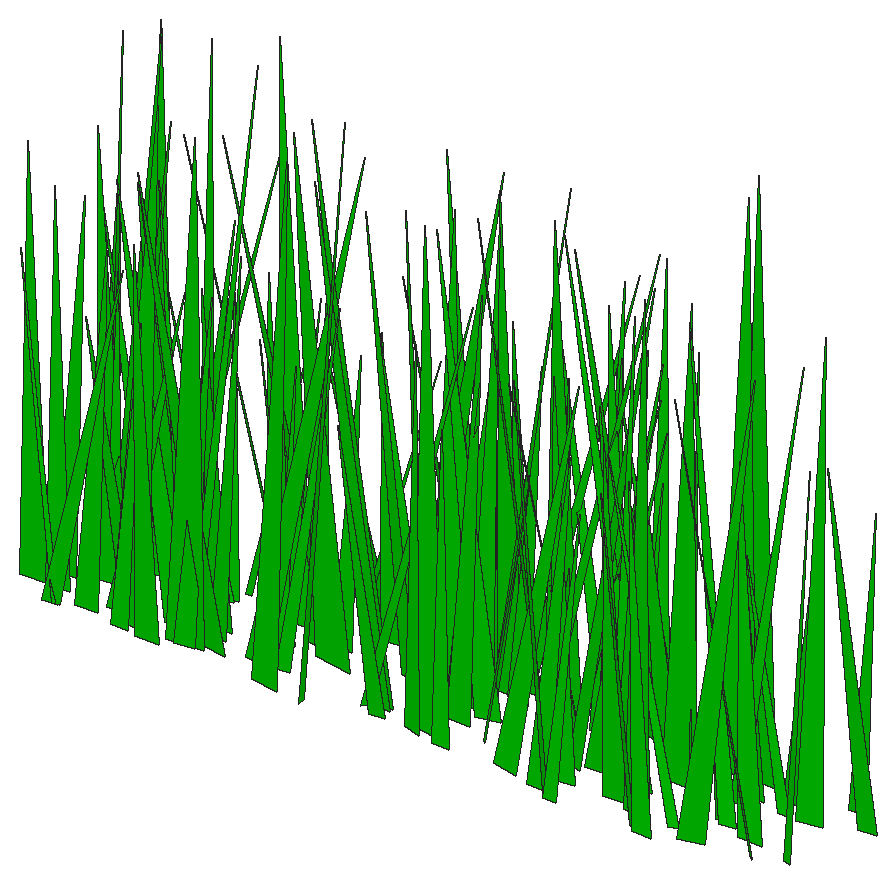
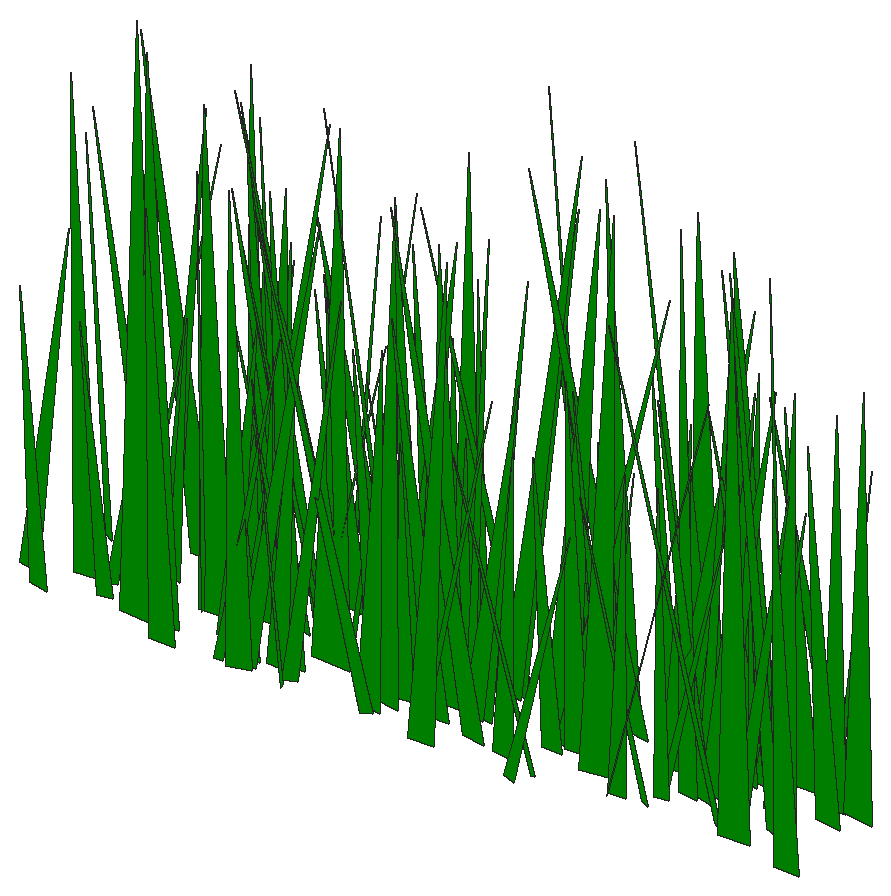
# SketchUp Ruby script. Lengths in inches.
U = 1.inch
M = Sketchup.active_model
def pt(a) = Geom::Point3d.new(a.map { |v| v * U })
def face(e, loops, mat)
  f = e.add_face(loops[0].map { |a| pt(a) })
  loops[1..].each { |l| e.add_face(l.map { |a| pt(a) }).erase! }
  f.material = f.back_material = mat if mat
  f
end
# faces: each face lists its corners as indices into pts; further lists are holes
def faces(e, pts, list, mat = nil) = list.each { |f| face(e, (f[0].is_a?(Array) ? f : [f]).map { |l| l.map { |i| pts[i] } }, mat) }
# xy, xz, yz: faces in a plane at the given z, y or x. An outline is a flat list of corners, or four numbers for a rectangle; further outlines are holes
def ring(l) = l.size == 4 ? [[l[0], l[1]], [l[2], l[1]], [l[2], l[3]], [l[0], l[3]]] : l.each_slice(2).to_a
def flat(e, list, mat, &to3) = list.each { |f| face(e, (f[0].is_a?(Array) ? f : [f]).map { |l| ring(l).map { |u, v| to3.(u, v) } }, mat) }
def xy(e, z, list, mat = nil) = flat(e, list, mat) { |x, y| [x, y, z] }
def xz(e, y, list, mat = nil) = flat(e, list, mat) { |x, z| [x, y, z] }
def yz(e, x, list, mat = nil) = flat(e, list, mat) { |y, z| [x, y, z] }
def lines(e, pts, list) = list.each { |a, b| e.add_line(pt(pts[a]), pt(pts[b])) }
# prism: a flat outline (further loops are holes) pulled along v
def prism(e, loops, v, mat = nil)
  f = face(e, loops, mat); d = Geom::Vector3d.new(v.map { |x| x * U })
  f.pushpull(f.normal.samedirection?(d) ? d.length : -d.length)
end
def box(e, o, s, mat = nil) = prism(e, [[o, [o[0] + s[0], o[1], o[2]], [o[0] + s[0], o[1] + s[1], o[2]], [o[0], o[1] + s[1], o[2]]]], [0, 0, s[2]], mat)
def at(x, y, z, deg = 0) = Geom::Transformation.translation(pt([x, y, z])) * Geom::Transformation.rotation(ORIGIN, Z_AXIS, deg.degrees)
def axes(o, x, y, z) = Geom::Transformation.new([*x, 0, *y, 0, *z, 0, *pt(o).to_a, 1])
def part(name) = M.definitions.add(name)
# library, detail: a bought-in or finely detailed component or shape, given as its bounding box
def library(name, o, s) = part(name).tap { |d| box(d.entities, o, s) }
def detail(e, o, s) = box(e.add_group.entities, o, s)
def put(e, d, t, mat = nil) = e.add_instance(d, t).tap { |i| i.material = mat if mat }
def group(e, t, mat = nil) = e.add_group.tap { |g| g.transformation = t; g.material = mat if mat }.entities
root = M.entities
M.materials.add("[Color G06]").color = [0, 204, 0]
c1 = part("fur_instance\#9")
p = [[0.8125,0,1.79],[0.67,-0.02,1.48],[0,-0.11,0],[0,0.11,0]]
faces(c1.entities,p,[[0,1,2,3]])
put(root,c1,axes([66.83,16.76,4.28],[0.70712,0.57146,2.51292],[4.40533,-0.11555,0.24948],[-0.46309,-0.22659,6.2104]),"[Color G06]")
put(root,c1,axes([66.57,20.13,4.28],[1.66976,-0.51159,0.9789],[-3.70784,-0.23812,-0.16793],[-0.37482,0.07652,6.02204]),"[Color G06]")
put(root,c1,axes([68.1,16.04,4.28],[-3.45503,0.0613,1.28299],[0.39453,0.4961,-0.34967],[0.88006,0.01826,5.19367]),"[Color G06]")
put(root,c1,axes([67.29,17.46,4.28],[1.39054,0.5281,0.88835],[3.81428,-0.19942,0.2814],[-0.3833,-0.06857,6.02306]),"[Color G06]")
put(root,c1,axes([67.625,16.76,4.28],[-2.06098,0.45345,2.2384],[3.47569,0.3112,-0.0935],[0.85835,-0.17136,5.75321]),"[Color G06]")
put(root,c1,axes([68.6,17.85,4.28],[-0.6422,0.67546,0.37884],[4.84661,0.08792,0.34379],[-0.19506,-0.03922,7.29482]),"[Color G06]")
put(root,c1,axes([69.18,18.85,4.28],[-3.10384,0.27643,0.94882],[2.03869,0.43579,0.31188],[0.42019,-0.07246,5.49549]),"[Color G06]")
put(root,c1,axes([68.12,18.32,4.28],[5.07652,0.17543,3.19542],[1.41724,-0.76243,-0.22092],[-2.036,-0.0933,7.81363]),"[Color G06]")
put(root,c1,axes([68.54,17.97,4.28],[-1.98125,0.30032,1.94706],[2.31896,0.30769,-0.18089],[0.97875,-0.12107,4.36994]),"[Color G06]")
put(root,c1,axes([68.08,18.76,4.28],[4.81626,0.3761,2.3505],[2.78245,-0.69993,0.12995],[-1.41619,-0.09614,8.24905]),"[Color G06]")
put(root,c1,axes([68.7,19.68,4.28],[-1.91202,-0.68423,2.93449],[-5.19419,0.29703,0.39628],[0.97564,0.24046,7.86064]),"[Color G06]")
put(root,c1,axes([67.97,16.03,4.28],[3.31947,-0.34025,0.11832],[-2.4411,-0.46283,0.08668],[-0.02942,0.01305,6.15668]),"[Color G06]")
put(root,c1,axes([69.99,16.875,4.28],[-1.54754,-0.3765,0.40529],[-2.71341,0.21421,-0.284],[-0.03089,0.04597,4.64251]),"[Color G06]")
put(root,c1,axes([68.92,16.34,4.28],[1.95061,-0.46199,1.20205],[-3.38606,-0.27757,0.01875],[-0.39701,0.09755,5.74603]),"[Color G06]")
put(root,c1,axes([70.57,18.18,4.28],[-1.25331,-0.60584,0.50701],[-4.35782,0.17399,-0.17996],[-0.02202,0.0501,6.75578]),"[Color G06]")
put(root,c1,axes([71.33,17.18,4.28],[-3.00174,0.47818,0.48813],[3.44352,0.41813,0.24732],[0.09014,-0.04948,6.80686]),"[Color G06]")
put(root,c1,axes([70.125,17.08,4.28],[2.45799,-0.13614,1.39658],[-0.94327,-0.36651,-0.39592],[-0.96778,0.01145,3.93296]),"[Color G06]")
put(root,c1,axes([69.69,16.93,4.28],[4.64119,0.29399,2.06947],[2.19856,-0.66971,-0.08469],[-1.23632,-0.08731,7.61827]),"[Color G06]")
put(root,c1,axes([71.68,19,4.28],[-3.04482,0.11833,0.27712],[0.85341,0.42509,0.0941],[0.16164,-0.01541,4.72318]),"[Color G06]")
put(root,c1,axes([70.22,16.12,4.28],[2.28875,-0.28835,1.54865],[-2.22991,-0.32907,0.32314],[-0.61407,0.12023,4.59871]),"[Color G06]")
put(root,c1,axes([70.4,16.36,4.28],[0.41336,0.76781,1.30806],[5.57291,-0.05332,-0.33883],[0.16343,-0.12399,8.24559]),"[Color G06]")
put(root,c1,axes([69.57,16.8,4.28],[3.12255,-0.33232,0.11448],[-2.38433,-0.43528,0.12169],[-0.01147,0.01551,5.8695]),"[Color G06]")
put(root,c1,axes([71.23,16.02,4.28],[-1.27828,-0.49619,2.17206],[-3.82734,0.18396,-0.20394],[0.35344,0.19749,5.64718]),"[Color G06]")
put(root,c1,axes([72.89,19.86,4.28],[-4.76011,-0.05072,0.37207],[-0.35967,0.66462,0.12951],[0.25479,-0.00942,7.13391]),"[Color G06]")
put(root,c1,axes([69.45,19.4,4.28],[4.95223,0.23128,0.28465],[1.64836,-0.69056,0.39613],[-0.26459,0.02665,7.79548]),"[Color G06]")
put(root,c1,axes([71.15,18.57,4.28],[4.44586,0.42134,3.46668],[3.31303,-0.67304,-0.09391],[-1.87979,-0.18969,8.03344]),"[Color G06]")
put(root,c1,axes([70.68,18.49,4.28],[2.95516,0.40171,0.98328],[2.89801,-0.41935,0.22517],[-0.57728,-0.04876,6.16395]),"[Color G06]")
put(root,c1,axes([72.17,16.57,4.28],[-4.27976,0.16657,2.23807],[1.29906,0.62802,0.17965],[1.40771,-0.07315,6.63845]),"[Color G06]")
put(root,c1,axes([71.625,19.125,4.28],[2.29948,-0.25988,1.81629],[-2.00537,-0.34765,-0.0431],[-0.96369,0.10332,4.42357]),"[Color G06]")
put(root,c1,axes([72.97,16.66,4.28],[-3.17325,-0.55502,0.35688],[-3.9826,0.44325,0.08797],[0.19492,0.02091,7.60738]),"[Color G06]")
put(root,c1,axes([72.35,17.69,4.28],[-0.24066,-0.53785,0.10636],[-3.85756,0.03345,-0.06409],[-0.03838,0.01028,5.77556]),"[Color G06]")
put(root,c1,axes([72.66,19.74,4.28],[-2.08194,0.32799,1.85752],[2.54477,0.30969,0.08937],[0.77544,-0.13569,4.69386]),"[Color G06]")
put(root,c1,axes([72.18,16.46,4.28],[1.4281,-0.80026,0.17463],[-5.73713,-0.19954,-0.23835],[-0.18299,0.01043,8.83551]),"[Color G06]")
put(root,c1,axes([72.2,16.4,4.28],[2.43363,-0.406,1.10403],[-2.96298,-0.34625,-0.03765],[-0.49343,0.07674,5.6713]),"[Color G06]")
put(root,c1,axes([71.8,19.625,4.28],[2.9454,0.17528,0.18578],[1.24841,-0.41066,0.29747],[-0.19229,0.01876,4.77698]),"[Color G06]")
put(root,c1,axes([72.62,17.29,4.28],[2.6975,0.39177,1.63323],[2.89485,-0.3937,0.16868],[-0.84107,-0.09855,5.81871]),"[Color G06]")
put(root,c1,axes([72.06,16.94,4.28],[6.03467,-0.12505,2.2423],[-0.92586,-0.86653,0.01481],[-1.4825,0.03216,9.11829]),"[Color G06]")
put(root,c1,axes([73.81,19.19,4.28],[-3.29736,0.66619,2.36389],[4.92298,0.4817,-0.25527],[1.04374,-0.16742,8.67199]),"[Color G06]")
put(root,c1,axes([75.51,18.51,4.28],[-4.78607,-0.3499,0.24867],[-2.50185,0.66756,0.34529],[0.25455,-0.01778,8.06924]),"[Color G06]")
put(root,c1,axes([74.37,18.27,4.28],[-2.78305,-0.16238,1.02207],[-1.16808,0.39908,0.17881],[0.67771,0.021,4.50537]),"[Color G06]")
put(root,c1,axes([74.34,17.85,4.28],[0.64409,-0.3519,1.03219],[-2.60627,-0.09499,-0.08755],[-0.22947,0.0912,3.89157]),"[Color G06]")
put(root,c1,axes([75.48,20.8,4.28],[-2.2374,-0.26843,0.12242],[-1.92497,0.31068,-0.33011],[-0.08219,0.03079,4.39891]),"[Color G06]")
put(root,c1,axes([74,18.4375,4.28],[3.44354,-0.17526,1.2215],[-1.23929,-0.49343,-0.32894],[-0.84368,0.00947,5.46883]),"[Color G06]")
put(root,c1,axes([74.45,17.625,4.28],[2.34333,-0.24978,1.31817],[-1.86168,-0.34187,-0.04904],[-0.72146,0.07089,4.408]),"[Color G06]")
put(root,c1,axes([74.93,18.59,4.28],[0.70413,0.48637,2.10076],[3.75822,-0.09787,-0.21083],[-0.12926,-0.19616,5.31386]),"[Color G06]")
put(root,c1,axes([75.91,18.05,4.28],[-1.93115,-0.76471,0.66967],[-5.48915,0.27232,0.36408],[0.37915,0.04757,8.68189]),"[Color G06]")
put(root,c1,axes([75.18,16.07,4.28],[-3.09751,-0.50765,4.07289],[-4.18001,0.49891,0.04245],[1.79081,0.28646,7.14383]),"[Color G06]")
put(root,c1,axes([75.52,18.91,4.28],[0.46261,0.44036,0.46927],[3.17326,-0.06365,-0.12606],[0.03836,-0.04502,4.76845]),"[Color G06]")
put(root,c1,axes([74.28,16.88,4.28],[4.42171,0.5679,0.29919],[4.07454,-0.61697,0.01815],[-0.15548,-0.01766,8.98453]),"[Color G06]")
put(root,c1,axes([75.0625,16.99,4.28],[3.69686,-0.2435,0.98505],[-1.78111,-0.5212,0.13095],[-0.55791,0.05043,6.10919]),"[Color G06]")
put(root,c1,axes([76.37,19.94,4.28],[0.1093,-0.41163,1.75668],[-3.1703,-0.025,-0.23224],[-0.21055,0.1627,4.40873]),"[Color G06]")
put(root,c1,axes([75.0625,20.29,4.28],[3.16739,0.1345,0.01271],[0.96247,-0.44044,-0.36675],[0.06337,-0.03308,4.93491]),"[Color G06]")
put(root,c1,axes([78.3,17.19,4.28],[-4.62122,-0.50231,1.73508],[-3.68936,0.65488,-0.17026],[0.84404,0.11228,8.75554]),"[Color G06]")
put(root,c1,axes([76.5,15.98,4.28],[5.92277,-0.007,2.76756],[-0.03278,-0.8653,-0.09468],[-1.85213,-0.00707,8.85183]),"[Color G06]")
put(root,c1,axes([78.25,17.08,4.28],[-3.75777,-0.52209,1.39761],[-3.81141,0.53063,-0.12025],[0.60469,0.1001,7.92721]),"[Color G06]")
put(root,c1,axes([77.95,18.72,4.28],[-3.90089,-0.35092,1.67875],[-2.55758,0.56209,0.22217],[1.02629,0.06694,6.93452]),"[Color G06]")
put(root,c1,axes([78.3,18.8125,4.28],[-2.59319,0.39094,0.74982],[2.83994,0.36208,0.25292],[0.21504,-0.06747,5.7021]),"[Color G06]")
put(root,c1,axes([78.78,20.39,4.28],[-3.70728,-0.16714,0.69156],[-1.22924,0.51874,-0.31723],[0.37386,0.04818,5.81456]),"[Color G06]")
put(root,c1,axes([78.56,16.6,4.28],[-1.42272,-0.37123,0.5573],[-2.6882,0.19637,-0.30287],[-0.00473,0.05918,4.50124]),"[Color G06]")
put(root,c1,axes([78.55,20.73,4.28],[-3.50452,0.47451,2.3814],[3.60945,0.50957,0.20115],[1.04408,-0.16888,7.29789]),"[Color G06]")
put(root,c1,axes([78.75,18.37,4.28],[-4.27028,-0.23829,2.61224],[-1.85445,0.63544,-0.11277],[1.5925,0.10099,6.87338]),"[Color G06]")
put(root,c1,axes([77.51,19.77,4.28],[4.0716,0.52637,0.80168],[3.7891,-0.5708,0.06604],[-0.42352,-0.04631,8.29789]),"[Color G06]")
put(root,c1,axes([79.16,18.73,4.28],[-0.19596,0.74073,0.1795],[5.31323,0.02741,-0.03564],[0.02827,-0.01661,7.94441]),"[Color G06]")
put(root,c1,axes([78.96,19.49,4.28],[1.89922,0.52007,0.85978],[3.77211,-0.26423,-0.25221],[-0.10904,-0.0822,6.25017]),"[Color G06]")
put(root,c1,axes([79.89,17.24,4.28],[-0.10028,0.38572,0.12762],[2.7637,0.01334,0.21871],[-0.14322,-0.01262,4.13106]),"[Color G06]")
put(root,c1,axes([77.95,16.91,4.28],[4.86652,-0.15825,0.0994],[-1.13191,-0.67831,-0.26951],[-0.10568,-0.02239,7.46367]),"[Color G06]")
put(root,c1,axes([79.76,16.6,4.28],[2.9254,0.30075,2.56144],[2.4657,-0.44131,-0.33802],[-1.22841,-0.16961,5.42147]),"[Color G06]")
put(root,c1,axes([80.96,18.31,4.28],[-3.4871,0.47923,1.24169],[3.49723,0.49144,0.15026],[0.52002,-0.09143,7.31586]),"[Color G06]")
put(root,c1,axes([80.14,18.54,4.28],[-0.48953,-0.34224,1.54934],[-2.65903,0.07194,-0.05118],[0.16641,0.14276,3.74001]),"[Color G06]")
put(root,c1,axes([80.21,16.71,4.28],[-1.7415,-0.66479,2.43086],[-4.97119,0.26555,0.38715],[0.81284,0.19974,7.57585]),"[Color G06]")
put(root,c1,axes([80.28,19.22,4.28],[-0.48854,0.37084,0.82968],[2.7061,0.07337,-0.20764],[0.23966,-0.07246,4.03579]),"[Color G06]")
put(root,c1,axes([80.6,19.7,4.28],[-2.38841,-0.57181,3.0749],[-4.50128,0.35458,-0.23542],[0.88656,0.25982,7.0885]),"[Color G06]")
put(root,c1,axes([80.04,18.18,4.28],[1.87539,-0.46685,0.23524],[-3.34032,-0.26241,-0.33937],[-0.27506,0.00363,5.72524]),"[Color G06]")
put(root,c1,axes([80.82,20.125,4.28],[0.77509,0.46156,2.4322],[3.636,-0.13456,0.34511],[-0.61944,-0.2123,5.06909]),"[Color G06]")
put(root,c1,axes([80.25,18.86,4.28],[3.58802,-0.46902,2.06485],[-3.44122,-0.52543,-0.35298],[-1.17456,0.10665,7.34183]),"[Color G06]")
put(root,c1,axes([80.44,17.71,4.28],[2.39596,0.5158,1.59152],[3.77602,-0.34891,0.29187],[-0.74697,-0.10928,6.58034]),"[Color G06]")
put(root,c1,axes([80.87,16.4,4.28],[-1.93517,0.3227,1.87901],[2.48042,0.29644,-0.14201],[0.88507,-0.12521,4.50635]),"[Color G06]")
put(root,c1,axes([80.95,19.57,4.28],[1.44458,0.42984,1.59528],[3.2542,-0.20118,-0.35545],[-0.22615,-0.1492,5.07537]),"[Color G06]")
put(root,c1,axes([82.72,18.52,4.28],[-4.99589,-0.16897,1.55281],[-1.19945,0.7115,0.2739],[1.05312,0.00879,7.67833]),"[Color G06]")
put(root,c1,axes([80.67,18.86,4.28],[5.76857,-0.0427,1.62556],[-0.26562,-0.81815,-0.36315],[-1.09826,-0.0264,8.62604]),"[Color G06]")
put(root,c1,axes([81.64,17.32,4.28],[2.75162,0.05827,0.6699],[0.41759,-0.38873,0.0532],[-0.44851,-0.00441,4.15932]),"[Color G06]")
put(root,c1,axes([83.35,20.3,4.28],[-3.80327,0.28017,1.01328],[2.0106,0.53815,-0.23572],[0.67364,-0.02444,6.42434]),"[Color G06]")
put(root,c1,axes([83.76,18.77,4.28],[-3.6137,-0.09377,0.42295],[-0.66177,0.50525,0.23726],[0.30708,-0.01461,5.48852]),"[Color G06]")
put(root,c1,axes([80.66,20.41,4.28],[4.93518,-0.20769,0.12616],[-1.49047,-0.68819,0.08941],[-0.06352,0.01139,7.70405]),"[Color G06]")
put(root,c1,axes([83.07,18.89,4.28],[0.65953,-0.81989,0.18193],[-5.87784,-0.09245,-0.26463],[-0.18956,0.01411,8.8387]),"[Color G06]")
put(root,c1,axes([83.21,18.69,4.28],[2.92807,0.25713,2.14442],[1.97707,-0.44362,0.08032],[-1.24497,-0.09974,5.17105]),"[Color G06]")
put(root,c1,axes([84.81,20.27,4.28],[-3.83725,-0.43927,0.96071],[-3.17896,0.53925,-0.0382],[0.48047,0.05965,7.41996]),"[Color G06]")
put(root,c1,axes([84.06,19.93,4.28],[-1.27921,0.39697,1.59861],[3.03298,0.17833,0.33443],[0.22152,-0.14922,4.65249]),"[Color G06]")
put(root,c1,axes([83.32,20.68,4.28],[3.01021,0.00056,1.22851],[-0.02631,-0.43483,0.16693],[-0.82157,0.01599,4.49588]),"[Color G06]")
put(root,c1,axes([83.92,19.64,4.28],[1.37466,-0.33207,1.08284],[-2.4471,-0.20141,-0.15589],[-0.45537,0.07992,4.10657]),"[Color G06]")
put(root,c1,axes([82.97,16.51,4.28],[2.58948,0.51195,0.27195],[3.67521,-0.36001,-0.31687],[0.06864,-0.03777,6.70716]),"[Color G06]")
put(root,c1,axes([84.67,16.09,4.28],[-3.86701,-0.14108,1.85733],[-1.08874,0.56345,-0.14689],[1.17583,0.05773,5.97225]),"[Color G06]")
put(root,c1,axes([83.75,19.67,4.28],[-2.83465,0.39367,4.1743],[3.53423,0.4683,0.28765],[1.81103,-0.29771,5.97233]),"[Color G06]")
put(root,c1,axes([84.6,16.91,4.28],[-1.9375,0.45712,2.46515],[3.59988,0.28724,0.20134],[0.71233,-0.2083,5.68759]),"[Color G06]")
put(root,c1,axes([85.56,20.5625,4.28],[-3.55911,0.13109,0.79367],[0.98171,0.49909,0.36383],[0.44949,-0.05203,5.48975]),"[Color G06]")
put(root,c1,axes([82.53,18.63,4.28],[5.77937,-0.15127,0.40328],[-1.07444,-0.80638,-0.35231],[-0.30852,-0.0254,8.78148]),"[Color G06]")
put(root,c1,axes([84.29,16.25,4.28],[1.28106,0.48821,0.22646],[3.50265,-0.17908,0.09021],[-0.10879,-0.01695,5.57115]),"[Color G06]")
put(root,c1,axes([84.65,18.86,4.28],[0.33108,0.54585,1.89562],[4.11477,-0.0431,-0.17972],[0.01907,-0.17764,5.86858]),"[Color G06]")
put(root,c1,axes([84.83,20.61,4.28],[-3.02833,0.45645,3.12242],[3.5567,0.47432,-0.25992],[1.55865,-0.1955,6.65974]),"[Color G06]")
put(root,c1,axes([84.74,20.0625,4.28],[2.26957,-0.20162,1.02817],[-1.49112,-0.32677,-0.00843],[-0.58333,0.05086,4.02187]),"[Color G06]")
put(root,c1,axes([86.59,17.83,4.28],[-5.09959,0.30971,1.15597],[2.22805,0.71866,-0.16307],[0.75296,-0.02897,8.31161]),"[Color G06]")
put(root,c1,axes([84.1,18.96,4.28],[3.40777,0.20427,0.35355],[1.45503,-0.47621,0.27998],[-0.29118,0.01104,5.53673]),"[Color G06]")
put(root,c1,axes([85.66,18.19,4.28],[-1.24913,0.66778,0.63902],[4.807,0.17463,0.02646],[0.09072,-0.05832,7.39665]),"[Color G06]")
put(root,c1,axes([84.9375,15.93,4.28],[2.5665,-0.2243,1.20085],[-1.70613,-0.36543,0.30437],[-0.56739,0.08426,4.51665]),"[Color G06]")
put(root,c1,axes([84.05,17.99,4.28],[4.34888,-0.05167,0.39297],[-0.36949,-0.60754,-0.04249],[-0.26439,-0.00085,6.52313]),"[Color G06]")
put(root,c1,axes([84.34,17.73,4.28],[4.83509,0.32462,1.20555],[2.34463,-0.68237,0.10231],[-0.75674,-0.04009,8.01971]),"[Color G06]")
put(root,c1,axes([86.05,19.5625,4.28],[-0.5762,-0.48828,0.1605],[-3.50083,0.07969,-0.22268],[-0.12966,0.01814,5.29907]),"[Color G06]")
put(root,c1,axes([85.68,18.02,4.28],[1.18613,-0.33878,0.43715],[-2.42536,-0.16878,-0.32592],[-0.32501,0.02311,4.02754]),"[Color G06]")
put(root,c1,axes([84.84,17.94,4.28],[3.47987,0.43395,0.51275],[3.10257,-0.48756,0.36746],[-0.41971,-0.00622,6.96757]),"[Color G06]")
put(root,c1,axes([86.28,17.03,4.28],[-0.02912,-0.51903,1.11117],[-3.79478,0.00182,-0.12473],[-0.07929,0.10374,5.5617]),"[Color G06]")
put(root,c1,axes([86.07,17.31,4.28],[4.50468,-0.18046,2.65432],[-1.42904,-0.66967,0.18732],[-1.66932,0.08632,7.00238]),"[Color G06]")
put(root,c1,axes([86.52,17.1,4.28],[2.90145,0.48191,2.26507],[3.66809,-0.42277,-0.16293],[-0.88613,-0.17212,6.74214]),"[Color G06]")
put(root,c1,axes([87.5625,16.15,4.28],[-3.16173,-0.12246,1.30847],[-0.86272,0.4574,0.26104],[0.89073,0.00834,4.89738]),"[Color G06]")
put(root,c1,axes([88.45,16.8125,4.28],[-3.48902,0.18691,0.47188],[1.34518,0.48826,0.00004],[0.29472,-0.01579,5.58617]),"[Color G06]")
put(root,c1,axes([87.26,16.72,4.28],[-3.09422,-0.51999,3.42894],[-4.09074,0.48298,0.16797],[1.56034,0.23506,7.24008]),"[Color G06]")
put(root,c1,axes([87.12,18.72,4.28],[1.13759,-0.73579,0.78585],[-5.3021,-0.15892,0.05204],[-0.07661,0.0727,8.06717]),"[Color G06]")
put(root,c1,axes([87.53,18.72,4.28],[-4.08344,0.03504,2.92995],[0.1897,0.63153,-0.27697],[1.96731,0.01183,6.10827]),"[Color G06]")
put(root,c1,axes([87.28,20.82,4.28],[2.49864,-0.49958,1.50712],[-3.65125,-0.36186,-0.25731],[-0.72132,0.10115,6.52303]),"[Color G06]")
put(root,c1,axes([88.01,15.99,4.28],[-2.33127,0.36715,1.2804],[2.66552,0.33986,-0.35405],[0.74918,-0.0667,5.24402]),"[Color G06]")
put(root,c1,axes([87.97,20.07,4.28],[-0.20407,0.81225,2.3447],[6.02907,0.03478,-0.21197],[0.2017,-0.21785,8.70847]),"[Color G06]")
put(root,c1,axes([88.59,20.16,4.28],[1.57908,0.78527,3.29591],[6.00283,-0.2422,0.20467],[-0.73616,-0.2905,8.73879]),"[Color G06]")
put(root,c1,axes([88.84,19.32,4.28],[-2.82528,0.00876,1.8751],[0.18514,0.42882,0.39305],[1.24246,-0.04398,4.2053]),"[Color G06]")
put(root,c1,axes([89.5,17.78,4.28],[-4.48541,0.2826,1.94353],[2.0548,0.64909,-0.24917],[1.25536,-0.05271,7.35206]),"[Color G06]")
put(root,c1,axes([89.21,17.9,4.28],[-1.79407,-0.25348,1.5995],[-2.03267,0.26011,-0.35744],[0.5639,0.13115,3.80041]),"[Color G06]")
put(root,c1,axes([89.13,19.42,4.28],[-0.46539,-0.39644,0.12555],[-2.84183,0.0653,0.15503],[0.11597,0.00921,4.30277]),"[Color G06]")
put(root,c1,axes([90.3,19.18,4.28],[-2.13727,0.22869,0.10581],[1.63304,0.29786,-0.27082],[0.16639,0.01406,4.0172]),"[Color G06]")
put(root,c1,axes([91.03,16.87,4.28],[-4.49991,-0.11977,0.94315],[-0.85912,0.63358,0.08642],[0.63075,0.0085,6.84632]),"[Color G06]")
put(root,c1,axes([88.97,18.87,4.28],[4.55141,-0.23704,1.34164],[-1.75516,-0.64364,0.23668],[-0.78414,0.06481,7.25752]),"[Color G06]")
put(root,c1,axes([90.5,17.48,4.28],[-1.69159,0.48982,0.99218],[3.54647,0.24282,-0.26443],[0.44944,-0.07246,5.82096]),"[Color G06]")
put(root,c1,axes([90.04,19.82,4.28],[1.14019,0.34564,1.08832],[2.58212,-0.15598,-0.35221],[-0.08159,-0.10612,4.06245]),"[Color G06]")
put(root,c1,axes([89.29,16.51,4.28],[3.8852,-0.53885,0.48924],[-3.86008,-0.54355,-0.29872],[-0.37314,0.01237,8.18436]),"[Color G06]")
put(root,c1,axes([91.125,19.22,4.28],[3.40572,-0.49028,2.41592],[-3.6846,-0.50261,-0.11458],[-1.18252,0.15405,7.31497]),"[Color G06]")
put(root,c1,axes([91.75,20.5,4.28],[1.39995,0.39608,0.82759],[2.86791,-0.20135,0.23341],[-0.38671,-0.0594,4.72704]),"[Color G06]")
put(root,c1,axes([92.6,19.81,4.28],[-1.99112,-0.42525,1.18288],[-3.1422,0.27757,-0.35142],[0.23031,0.11056,5.43197]),"[Color G06]")
put(root,c1,axes([91.96,17.22,4.28],[3.70249,0.18548,1.95343],[1.36715,-0.54553,0.16218],[-1.26824,-0.04659,5.87767]),"[Color G06]")
